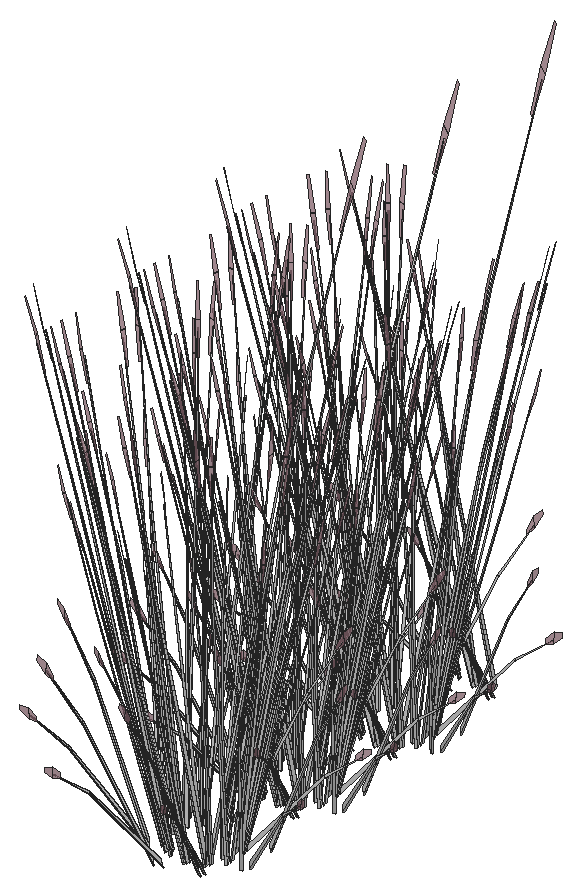
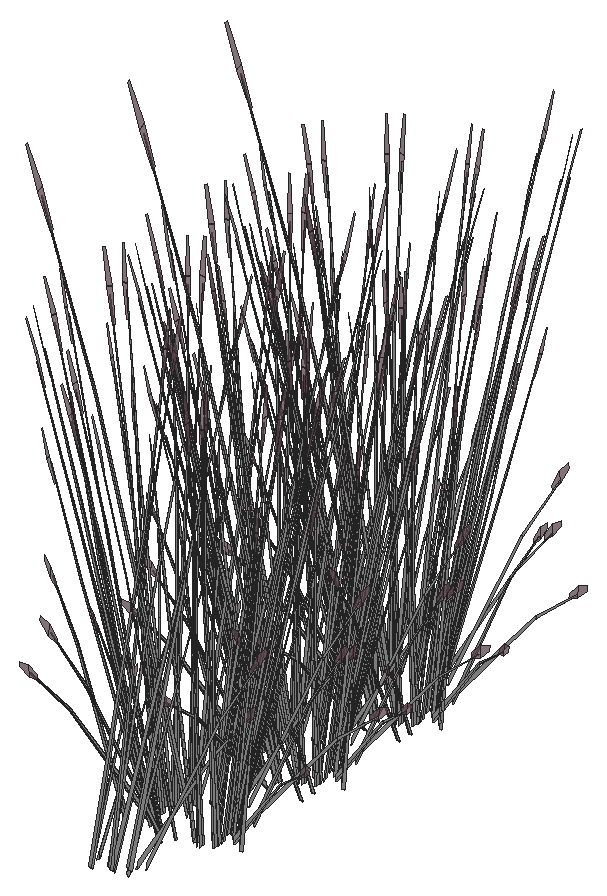
# SketchUp Ruby script. Lengths in inches.
U = 1.inch
M = Sketchup.active_model
def pt(a) = Geom::Point3d.new(a.map { |v| v * U })
def face(e, loops, mat)
  f = e.add_face(loops[0].map { |a| pt(a) })
  loops[1..].each { |l| e.add_face(l.map { |a| pt(a) }).erase! }
  f.material = f.back_material = mat if mat
  f
end
# faces: each face lists its corners as indices into pts; further lists are holes
def faces(e, pts, list, mat = nil) = list.each { |f| face(e, (f[0].is_a?(Array) ? f : [f]).map { |l| l.map { |i| pts[i] } }, mat) }
# xy, xz, yz: faces in a plane at the given z, y or x. An outline is a flat list of corners, or four numbers for a rectangle; further outlines are holes
def ring(l) = l.size == 4 ? [[l[0], l[1]], [l[2], l[1]], [l[2], l[3]], [l[0], l[3]]] : l.each_slice(2).to_a
def flat(e, list, mat, &to3) = list.each { |f| face(e, (f[0].is_a?(Array) ? f : [f]).map { |l| ring(l).map { |u, v| to3.(u, v) } }, mat) }
def xy(e, z, list, mat = nil) = flat(e, list, mat) { |x, y| [x, y, z] }
def xz(e, y, list, mat = nil) = flat(e, list, mat) { |x, z| [x, y, z] }
def yz(e, x, list, mat = nil) = flat(e, list, mat) { |y, z| [x, y, z] }
def lines(e, pts, list) = list.each { |a, b| e.add_line(pt(pts[a]), pt(pts[b])) }
# prism: a flat outline (further loops are holes) pulled along v
def prism(e, loops, v, mat = nil)
  f = face(e, loops, mat); d = Geom::Vector3d.new(v.map { |x| x * U })
  f.pushpull(f.normal.samedirection?(d) ? d.length : -d.length)
end
def box(e, o, s, mat = nil) = prism(e, [[o, [o[0] + s[0], o[1], o[2]], [o[0] + s[0], o[1] + s[1], o[2]], [o[0], o[1] + s[1], o[2]]]], [0, 0, s[2]], mat)
def at(x, y, z, deg = 0) = Geom::Transformation.translation(pt([x, y, z])) * Geom::Transformation.rotation(ORIGIN, Z_AXIS, deg.degrees)
def axes(o, x, y, z) = Geom::Transformation.new([*x, 0, *y, 0, *z, 0, *pt(o).to_a, 1])
def part(name) = M.definitions.add(name)
# library, detail: a bought-in or finely detailed component or shape, given as its bounding box
def library(name, o, s) = part(name).tap { |d| box(d.entities, o, s) }
def detail(e, o, s) = box(e.add_group.entities, o, s)
def put(e, d, t, mat = nil) = e.add_instance(d, t).tap { |i| i.material = mat if mat }
def group(e, t, mat = nil) = e.add_group.tap { |g| g.transformation = t; g.material = mat if mat }.entities
root = M.entities
M.materials.add("LightPink_Translucent").color = [144, 107, 117]
M.materials["LightPink_Translucent"].alpha = 0.75
M.materials.add("[_0053_Ivory_]").color = [200, 200, 200]
c1 = part("blade")
p = [[2.15,0.21,22],[0,0.17,0],[0.09,0.45,0],[2.18,0.31,22],[2.29,0.31,22],[0.38,0.45,0],
  [2.48,0.24,33],[2.49,0.24,33],[2.48,0.22,33]]
faces(c1.entities,p,[[0,1,2,3],[4,5,2,3],[6,3,4,7],[8,0,3,6]])
c2 = part("seeds")
p = [[0.3,-0.1,1.38],[-0.01,-0.03,1.59],[-0.01,-0.03,0.03],[0.14,-0.07,-0.07],[0.29,-0.03,3],[0.15,0.01,3.11]]
faces(c2.entities,p,[[0,1,2,3],[1,0,4,5]],"LightPink_Translucent")
c3 = part("blade with seeds")
put(c3.entities,c1,at(0,0,0))
put(c3.entities,c2,axes([2.4,0.25,30.99],[1.5799,-0.05474,1.17369],[-0.12525,1.92788,0.29478],[-0.07173,-0.02425,1.56792]))
put(root,c3,axes([631.55,280.53,256.37],[-0.0929,-0.08817,1.74944],[-0.61994,0.0559,-0.27667],[-0.09894,-0.21089,0.14031]),"[_0053_Ivory_]")
put(root,c3,axes([634.33,281.61,256.37],[-0.00586,-0.12516,1.74944],[-0.49517,-0.36172,-0.27667],[0.07656,-0.21927,0.14031]),"[_0053_Ivory_]")
put(root,c3,axes([634.2,281.16,256.36],[-0.06168,0.04803,1.77383],[-0.60432,-0.16205,-0.16761],[-0.02188,-0.20961,0.31391]),"[_0053_Ivory_]")
put(root,c3,axes([630.91,280.24,256.36],[-0.01133,0.07538,1.77383],[-0.55883,0.27355,-0.16761],[-0.16445,-0.13983,0.31391]),"[_0053_Ivory_]")
put(root,c3,axes([630.79,281.58,256.75],[0.67657,-0.16163,0.53763],[0.11742,0.63404,0.4433],[-0.15912,-0.18687,1.11249]),"[_0053_Ivory_]")
put(root,c3,axes([632.32,281.7,256.39],[0.59846,0.1644,0.48003],[-0.20464,0.54049,0.3958],[-0.03596,-0.21255,0.9933]),"[_0053_Ivory_]")
put(root,c3,axes([632.49,281.89,256.6875],[-0.59433,0.29278,-0.1216],[-0.29207,-0.51964,-0.67495],[-0.07842,-0.21898,1.02557]),"[_0053_Ivory_]")
put(root,c3,axes([633.72,282.55,256.6875],[-0.6675,-0.03116,-0.1216],[0.01824,-0.58993,-0.67495],[0.04637,-0.2272,1.02557]),"[_0053_Ivory_]")
put(root,c3,axes([632.48,281.65,256.38],[0.44753,-0.21372,0.0643],[0.21905,0.38973,0.50621],[-0.04322,-0.1718,0.77189]),"[_0053_Ivory_]")
put(root,c3,axes([630.94,281.71,256.38],[0.27604,-0.39948,0.0643],[0.39309,0.23258,0.50621],[-0.12709,-0.12808,0.77189]),"[_0053_Ivory_]")
put(root,c3,axes([632.31,282.09,256.7],[-0.1831,0.48359,0.35414],[-0.53419,-0.14105,-0.4572],[-0.04898,-0.1947,0.87481]),"[_0053_Ivory_]")
put(root,c3,axes([633.68,282.3,256.39],[0.43249,0.42907,0.48003],[-0.45929,0.37004,0.3958],[0.07978,-0.2013,0.9933]),"[_0053_Ivory_]")
put(root,c3,axes([631.07,281.67,257.08],[-0.40534,0.60286,-0.13619],[-0.58702,-0.34732,-0.75594],[-0.20405,-0.17032,1.14864]),"[_0053_Ivory_]")
put(root,c3,axes([633.84,282.34,256.38],[0.49911,0.0293,0.0643],[-0.01368,0.44245,0.50621],[0.05223,-0.16948,0.77189]),"[_0053_Ivory_]")
put(root,c3,axes([633.46,282.64,256.7],[-0.41095,0.33109,0.35414],[-0.38901,-0.37805,-0.4572],[0.05919,-0.19208,0.87481]),"[_0053_Ivory_]")
put(root,c3,axes([629.51,281.5,256.37],[-0.13068,-0.00444,1.74944],[-0.41604,0.44388,-0.27667],[-0.22198,-0.0907,0.14031]),"[_0053_Ivory_]")
put(root,c3,axes([634.45,283.71,256.6875],[-0.56181,-0.34675,-0.1216],[0.32367,-0.50216,-0.67495],[0.15873,-0.17455,1.02557]),"[_0053_Ivory_]")
put(root,c3,axes([631.03,282.17,256.7],[0.0938,0.50652,0.35414],[-0.53623,0.13375,-0.4572],[-0.14403,-0.14515,0.87481]),"[_0053_Ivory_]")
put(root,c3,axes([629.42,282.5,256.75],[0.50157,-0.46409,0.53763],[0.43258,0.49285,0.4433],[-0.23532,-0.08561,1.11249]),"[_0053_Ivory_]")
put(root,c3,axes([635.83,283.56,256.36],[-0.07933,-0.00478,1.77383],[-0.32942,-0.51175,-0.16761],[0.13229,-0.16826,0.31391]),"[_0053_Ivory_]")
put(root,c3,axes([629.65,282.5,256.38],[0.03058,-0.47819,0.0643],[0.4618,0.01311,0.50621],[-0.1769,-0.05004,0.77189]),"[_0053_Ivory_]")
put(root,c3,axes([634.18,283.66,256.7],[-0.52868,0.08987,0.35414],[-0.1396,-0.51376,-0.4572],[0.1515,-0.13799,0.87481]),"[_0053_Ivory_]")
put(root,c3,axes([634.66,283.58,256.38],[0.41695,0.26447,0.0643],[-0.24275,0.37662,0.50621],[0.13368,-0.12176,0.77189]),"[_0053_Ivory_]")
put(root,c3,axes([634.54,283.47,256.39],[0.15063,0.57876,0.48003],[-0.59087,0.10045,0.3958],[0.17414,-0.13612,0.9933]),"[_0053_Ivory_]")
put(root,c3,axes([636.13,284.17,256.37],[0.08428,-0.09579,1.74944],[-0.10787,-0.58756,-0.27667],[0.21147,-0.1114,0.14031]),"[_0053_Ivory_]")
put(root,c3,axes([629.01,281.875,256.36],[0.04503,0.06276,1.77383],[-0.21706,0.56413,-0.16761],[-0.21983,0.00408,0.31391]),"[_0053_Ivory_]")
put(root,c3,axes([629.96,282.86,256.7],[0.34557,0.39372,0.35414],[-0.39459,0.37271,-0.4572],[-0.20048,-0.05671,0.87481]),"[_0053_Ivory_]")
put(root,c3,axes([629.87,282.61,256.6875],[-0.03252,0.63953,-0.1216],[-0.61574,-0.01748,-0.67495],[-0.23714,-0.04442,1.02557]),"[_0053_Ivory_]")
put(root,c3,axes([634.47,285.0625,256.6875],[-0.30559,-0.56943,-0.1216],[0.54237,-0.27983,-0.67495],[0.22856,-0.07513,1.02557]),"[_0053_Ivory_]")
put(root,c3,axes([634.26,284.89,256.7],[-0.50475,-0.17543,0.35414],[0.14722,-0.5118,-0.4572],[0.20322,-0.04693,0.87481]),"[_0053_Ivory_]")
put(root,c3,axes([628.98,283.95,256.39],[0.17159,-0.57338,0.48003],[0.56413,0.19607,0.3958],[-0.22185,0.03446,0.9933]),"[_0053_Ivory_]")
put(root,c3,axes([628.93,283.8,256.38],[-0.22307,-0.42878,0.0643],[0.40677,-0.20987,0.50621],[-0.17931,0.04141,0.77189]),"[_0053_Ivory_]")
put(root,c3,axes([634.72,285.05,256.38],[0.22307,0.42878,0.0643],[-0.40677,0.20987,0.50621],[0.17931,-0.04141,0.77189]),"[_0053_Ivory_]")
put(root,c3,axes([634.68,284.9,256.39],[-0.17159,0.57338,0.48003],[-0.56413,-0.19607,0.3958],[0.22185,-0.03446,0.9933]),"[_0053_Ivory_]")
put(root,c3,axes([629.39,283.96,256.7],[0.50475,0.17543,0.35414],[-0.14722,0.5118,-0.4572],[-0.20322,0.04693,0.87481]),"[_0053_Ivory_]")
put(root,c3,axes([635.6875,286.75,256.36],[-0.05492,-0.05505,1.77383],[0.12013,-0.59013,-0.16761],[0.21632,-0.0377,0.31391]),"[_0053_Ivory_]")
put(root,c3,axes([628.54,284.36,256.37],[-0.09918,0.08165,1.74944],[0.00844,0.59653,-0.27667],[-0.22734,0.07758,0.14031]),"[_0053_Ivory_]")
put(root,c3,axes([629.18,283.79,256.6875],[0.30559,0.56943,-0.1216],[-0.54237,0.27983,-0.67495],[-0.22856,0.07513,1.02557]),"[_0053_Ivory_]")
put(root,c3,axes([633.79,286.24,256.6875],[0.03252,-0.63953,-0.1216],[0.61574,0.01748,-0.67495],[0.23714,0.04442,1.02557]),"[_0053_Ivory_]")
put(root,c3,axes([633.69,285.99,256.7],[-0.34557,-0.39372,0.35414],[0.39459,-0.37271,-0.4572],[0.20048,0.05671,0.87481]),"[_0053_Ivory_]")
put(root,c3,axes([631.55,290.36,256.37],[-0.0929,-0.08817,1.74944],[-0.61994,0.0559,-0.27667],[-0.09894,-0.21089,0.14031]),"[_0053_Ivory_]")
put(root,c3,axes([634.32,285.86,256.37],[0.13029,-0.01064,1.74944],[0.35737,-0.48855,-0.27667],[0.23175,0.06449,0.14031]),"[_0053_Ivory_]")
put(root,c3,axes([629.11,285.38,256.39],[-0.15063,-0.57876,0.48003],[0.59087,-0.10045,0.3958],[-0.17414,0.13612,0.9933]),"[_0053_Ivory_]")
put(root,c3,axes([629,285.27,256.38],[-0.41695,-0.26447,0.0643],[0.24275,-0.37662,0.50621],[-0.13368,0.12176,0.77189]),"[_0053_Ivory_]")
put(root,c3,axes([634.33,291.45,256.37],[-0.00586,-0.12516,1.74944],[-0.49517,-0.36172,-0.27667],[0.07656,-0.21927,0.14031]),"[_0053_Ivory_]")
put(root,c3,axes([634.2,291,256.36],[-0.06168,0.04803,1.77383],[-0.60432,-0.16205,-0.16761],[-0.02188,-0.20961,0.31391]),"[_0053_Ivory_]")
put(root,c3,axes([629.48,285.1875,256.7],[0.52868,-0.08987,0.35414],[0.1396,0.51376,-0.4572],[-0.1515,0.13799,0.87481]),"[_0053_Ivory_]")
put(root,c3,axes([630.91,290.08,256.36],[-0.01133,0.07538,1.77383],[-0.55883,0.27355,-0.16761],[-0.16445,-0.13983,0.31391]),"[_0053_Ivory_]")
put(root,c3,axes([627.4375,284.96,256.36],[0.07751,0.01687,1.77383],[0.23978,0.55562,-0.16761],[-0.15867,0.14583,0.31391]),"[_0053_Ivory_]")
put(root,c3,axes([630.79,291.41,256.75],[0.67657,-0.16163,0.53763],[0.11742,0.63404,0.4433],[-0.15912,-0.18687,1.11249]),"[_0053_Ivory_]")
put(root,c3,axes([634.01,286.35,256.38],[-0.03058,0.47819,0.0643],[-0.4618,-0.01311,0.50621],[0.1769,0.05004,0.77189]),"[_0053_Ivory_]")
put(root,c3,axes([632.32,291.53,256.39],[0.59846,0.1644,0.48003],[-0.20464,0.54049,0.3958],[-0.03596,-0.21255,0.9933]),"[_0053_Ivory_]")
put(root,c3,axes([632.49,291.73,256.6875],[-0.59433,0.29278,-0.1216],[-0.29207,-0.51964,-0.67495],[-0.07842,-0.21898,1.02557]),"[_0053_Ivory_]")
put(root,c3,axes([634.05,286.2,256.39],[-0.44783,0.41436,0.48003],[-0.38623,-0.44004,0.3958],[0.21011,0.07643,0.9933]),"[_0053_Ivory_]")
put(root,c3,axes([633.72,292.38,256.6875],[-0.6675,-0.03116,-0.1216],[0.01824,-0.58993,-0.67495],[0.04637,-0.2272,1.02557]),"[_0053_Ivory_]")
put(root,c3,axes([632.48,291.49,256.38],[0.44753,-0.21372,0.0643],[0.21905,0.38973,0.50621],[-0.04322,-0.1718,0.77189]),"[_0053_Ivory_]")
put(root,c3,axes([628.28,286.65,257.3],[0.53595,0.16786,-0.06488],[-0.16486,0.51664,-0.29416],[-0.08766,0.07844,0.97024]),"[_0053_Ivory_]")
put(root,c3,axes([632.625,286.68,256.7],[-0.0938,-0.50652,0.35414],[0.53623,-0.13375,-0.4572],[0.14403,0.14515,0.87481]),"[_0053_Ivory_]")
put(root,c3,axes([630.94,291.55,256.38],[0.27604,-0.39948,0.0643],[0.39309,0.23258,0.50621],[-0.12709,-0.12808,0.77189]),"[_0053_Ivory_]")
put(root,c3,axes([632.98,283.76,256.13],[-0.52482,-0.32674,1.38283],[0.55416,-0.50872,0.59665],[0.16933,0.30658,1.33663]),"[_0053_Ivory_]")
put(root,c3,axes([629.2,285.14,256.6875],[0.56181,0.34675,-0.1216],[-0.32367,0.50216,-0.67495],[-0.15873,0.17455,1.02557]),"[_0053_Ivory_]")
put(root,c3,axes([632.57,286.9375,256.6875],[0.36191,-0.53827,-0.1216],[0.52412,0.3101,-0.67495],[0.18219,0.15207,1.02557]),"[_0053_Ivory_]")
put(root,c3,axes([632.31,291.93,256.7],[-0.1831,0.48359,0.35414],[-0.53419,-0.14105,-0.4572],[-0.04898,-0.1947,0.87481]),"[_0053_Ivory_]")
put(root,c3,axes([633.68,292.13,256.39],[0.43249,0.42907,0.48003],[-0.45929,0.37004,0.3958],[0.07978,-0.2013,0.9933]),"[_0053_Ivory_]")
put(root,c3,axes([631.07,291.51,257.08],[-0.40534,0.60286,-0.13619],[-0.58702,-0.34732,-0.75594],[-0.20405,-0.17032,1.14864]),"[_0053_Ivory_]")
put(root,c3,axes([633.84,292.17,256.38],[0.49911,0.0293,0.0643],[-0.01368,0.44245,0.50621],[0.05223,-0.16948,0.77189]),"[_0053_Ivory_]")
put(root,c3,axes([630.1875,286.21,256.7],[0.41095,-0.33109,0.35414],[0.38901,0.37805,-0.4572],[-0.05919,0.19208,0.87481]),"[_0053_Ivory_]")
put(root,c3,axes([632.1,287.39,256.36],[0.0018,-0.07613,1.77383],[0.52048,-0.3359,-0.16761],[0.18079,0.11989,0.31391]),"[_0053_Ivory_]")
put(root,c3,axes([633.46,292.47,256.7],[-0.41095,0.33109,0.35414],[-0.38901,-0.37805,-0.4572],[0.05919,-0.19208,0.87481]),"[_0053_Ivory_]")
put(root,c3,axes([629.82,286.51,256.38],[-0.49911,-0.0293,0.0643],[0.01368,-0.44245,0.50621],[-0.05223,0.16948,0.77189]),"[_0053_Ivory_]")
put(root,c3,axes([629.98,286.55,256.39],[-0.43249,-0.42907,0.48003],[0.45929,-0.37004,0.3958],[-0.07978,0.2013,0.9933]),"[_0053_Ivory_]")
put(root,c3,axes([631.34,286.76,256.7],[0.1831,-0.48359,0.35414],[0.53419,0.14105,-0.4572],[0.04898,0.1947,0.87481]),"[_0053_Ivory_]")
put(root,c3,axes([629.51,291.34,256.37],[-0.13068,-0.00444,1.74944],[-0.41604,0.44388,-0.27667],[-0.22198,-0.0907,0.14031]),"[_0053_Ivory_]")
put(root,c3,axes([634.45,293.54,256.6875],[-0.56181,-0.34675,-0.1216],[0.32367,-0.50216,-0.67495],[0.15873,-0.17455,1.02557]),"[_0053_Ivory_]")
put(root,c3,axes([632.71,287.14,256.38],[-0.27604,0.39948,0.0643],[-0.39309,-0.23258,0.50621],[0.12709,0.12808,0.77189]),"[_0053_Ivory_]")
put(root,c3,axes([632.06,288.48,257.3],[0.4197,-0.36076,-0.06488],[0.38456,0.39511,-0.29416],[0.02707,0.11196,0.97024]),"[_0053_Ivory_]")
put(root,c3,axes([632.82,287.02,256.39],[-0.60408,0.14432,0.48003],[-0.10484,-0.56611,0.3958],[0.14207,0.16684,0.9933]),"[_0053_Ivory_]")
put(root,c3,axes([631.03,292.01,256.7],[0.0938,0.50652,0.35414],[-0.53623,0.13375,-0.4572],[-0.14403,-0.14515,0.87481]),"[_0053_Ivory_]")
put(root,c3,axes([629.42,292.34,256.75],[0.50157,-0.46409,0.53763],[0.43258,0.49285,0.4433],[-0.23532,-0.08561,1.11249]),"[_0053_Ivory_]")
put(root,c3,axes([635.83,293.39,256.36],[-0.07933,-0.00478,1.77383],[-0.32942,-0.51175,-0.16761],[0.13229,-0.16826,0.31391]),"[_0053_Ivory_]")
put(root,c3,axes([631.18,287.2,256.38],[-0.44753,0.21372,0.0643],[-0.21905,-0.38973,0.50621],[0.04322,0.1718,0.77189]),"[_0053_Ivory_]")
put(root,c3,axes([628.56,286.58,256.37],[-0.0151,0.12444,1.74944],[0.42844,0.43292,-0.27667],[-0.11216,0.20472,0.14031]),"[_0053_Ivory_]")
put(root,c3,axes([629.93,286.3,257.05],[0.6675,0.03116,-0.13498],[-0.01824,0.58993,-0.74919],[-0.04637,0.2272,1.13838]),"[_0053_Ivory_]")
put(root,c3,axes([631.16,286.96,256.6875],[0.59433,-0.29278,-0.1216],[0.29207,0.51964,-0.67495],[0.07842,0.21898,1.02557]),"[_0053_Ivory_]")
put(root,c3,axes([631.33,287.15,256.72],[-0.59846,-0.1644,0.53283],[0.20464,-0.54049,0.43934],[0.03596,0.21255,1.10256]),"[_0053_Ivory_]")
put(root,c3,axes([629.65,292.34,256.38],[0.03058,-0.47819,0.0643],[0.4618,0.01311,0.50621],[-0.1769,-0.05004,0.77189]),"[_0053_Ivory_]")
put(root,c3,axes([634.18,293.5,256.7],[-0.52868,0.08987,0.35414],[-0.1396,-0.51376,-0.4572],[0.1515,-0.13799,0.87481]),"[_0053_Ivory_]")
put(root,c3,axes([628.51,287.86,256.36],[0.0689,-0.03797,1.77383],[0.5695,0.25254,-0.16761],[-0.01338,0.21027,0.31391]),"[_0053_Ivory_]")
put(root,c3,axes([634.66,293.42,256.38],[0.41695,0.26447,0.0643],[-0.24275,0.37662,0.50621],[0.13368,-0.12176,0.77189]),"[_0053_Ivory_]")
put(root,c3,axes([634.54,293.3,256.39],[0.15063,0.57876,0.48003],[-0.59087,0.10045,0.3958],[0.17414,-0.13612,0.9933]),"[_0053_Ivory_]")
put(root,c3,axes([636.13,294.01,256.37],[0.08428,-0.09579,1.74944],[-0.10787,-0.58756,-0.27667],[0.21147,-0.1114,0.14031]),"[_0053_Ivory_]")
put(root,c3,axes([629.01,291.71,256.36],[0.04503,0.06276,1.77383],[-0.21706,0.56413,-0.16761],[-0.21983,0.00408,0.31391]),"[_0053_Ivory_]")
put(root,c3,axes([629.96,292.69,256.7],[0.34557,0.39372,0.35414],[-0.39459,0.37271,-0.4572],[-0.20048,-0.05671,0.87481]),"[_0053_Ivory_]")
put(root,c3,axes([631.02,288.125,256.37],[0.07699,0.10127,1.74944],[0.6213,0.03978,-0.27667],[0.06248,0.22333,0.14031]),"[_0053_Ivory_]")
put(root,c3,axes([629.87,292.44,256.6875],[-0.03252,0.63953,-0.1216],[-0.61574,-0.01748,-0.67495],[-0.23714,-0.04442,1.02557]),"[_0053_Ivory_]")
put(root,c3,axes([634.47,294.9,256.6875],[-0.30559,-0.56943,-0.1216],[0.54237,-0.27983,-0.67495],[0.22856,-0.07513,1.02557]),"[_0053_Ivory_]")
put(root,c3,axes([634.26,294.73,256.7],[-0.50475,-0.17543,0.35414],[0.14722,-0.5118,-0.4572],[0.20322,-0.04693,0.87481]),"[_0053_Ivory_]")
put(root,c3,axes([628.98,293.79,256.39],[0.17159,-0.57338,0.48003],[0.56413,0.19607,0.3958],[-0.22185,0.03446,0.9933]),"[_0053_Ivory_]")
put(root,c3,axes([628.93,293.64,256.38],[-0.22307,-0.42878,0.0643],[0.40677,-0.20987,0.50621],[-0.17931,0.04141,0.77189]),"[_0053_Ivory_]")
put(root,c3,axes([634.72,294.88,256.38],[0.22307,0.42878,0.0643],[-0.40677,0.20987,0.50621],[0.17931,-0.04141,0.77189]),"[_0053_Ivory_]")
put(root,c3,axes([634.68,294.73,256.39],[-0.17159,0.57338,0.48003],[-0.56413,-0.19607,0.3958],[0.22185,-0.03446,0.9933]),"[_0053_Ivory_]")
put(root,c3,axes([629.39,293.8,256.7],[0.50475,0.17543,0.35414],[-0.14722,0.5118,-0.4572],[-0.20322,0.04693,0.87481]),"[_0053_Ivory_]")
put(root,c3,axes([635.6875,296.59,256.36],[-0.05492,-0.05505,1.77383],[0.12013,-0.59013,-0.16761],[0.21632,-0.0377,0.31391]),"[_0053_Ivory_]")
put(root,c3,axes([628.54,294.19,256.37],[-0.09918,0.08165,1.74944],[0.00844,0.59653,-0.27667],[-0.22734,0.07758,0.14031]),"[_0053_Ivory_]")
put(root,c3,axes([629.18,293.625,256.6875],[0.30559,0.56943,-0.1216],[-0.54237,0.27983,-0.67495],[-0.22856,0.07513,1.02557]),"[_0053_Ivory_]")
put(root,c3,axes([633.79,296.08,256.6875],[0.03252,-0.63953,-0.1216],[0.61574,0.01748,-0.67495],[0.23714,0.04442,1.02557]),"[_0053_Ivory_]")
put(root,c3,axes([633.69,295.83,256.7],[-0.34557,-0.39372,0.35414],[0.39459,-0.37271,-0.4572],[0.20048,0.05671,0.87481]),"[_0053_Ivory_]")
put(root,c3,axes([631.55,300.66,256.37],[-0.0929,-0.08817,1.74944],[-0.61994,0.0559,-0.27667],[-0.09894,-0.21089,0.14031]),"[_0053_Ivory_]")
put(root,c3,axes([634.32,295.7,256.37],[0.13029,-0.01064,1.74944],[0.35737,-0.48855,-0.27667],[0.23175,0.06449,0.14031]),"[_0053_Ivory_]")
put(root,c3,axes([629.11,295.22,256.39],[-0.15063,-0.57876,0.48003],[0.59087,-0.10045,0.3958],[-0.17414,0.13612,0.9933]),"[_0053_Ivory_]")
put(root,c3,axes([629,295.11,256.38],[-0.41695,-0.26447,0.0643],[0.24275,-0.37662,0.50621],[-0.13368,0.12176,0.77189]),"[_0053_Ivory_]")
put(root,c3,axes([629.48,295.03,256.7],[0.52868,-0.08987,0.35414],[0.1396,0.51376,-0.4572],[-0.1515,0.13799,0.87481]),"[_0053_Ivory_]")
put(root,c3,axes([634.33,301.74,256.37],[-0.00586,-0.12516,1.74944],[-0.49517,-0.36172,-0.27667],[0.07656,-0.21927,0.14031]),"[_0053_Ivory_]")
put(root,c3,axes([634.2,301.29,256.36],[-0.06168,0.04803,1.77383],[-0.60432,-0.16205,-0.16761],[-0.02188,-0.20961,0.31391]),"[_0053_Ivory_]")
put(root,c3,axes([627.4375,294.8,256.36],[0.07751,0.01687,1.77383],[0.23978,0.55562,-0.16761],[-0.15867,0.14583,0.31391]),"[_0053_Ivory_]")
put(root,c3,axes([634.01,296.1875,256.38],[-0.03058,0.47819,0.0643],[-0.4618,-0.01311,0.50621],[0.1769,0.05004,0.77189]),"[_0053_Ivory_]")
put(root,c3,axes([634.05,296.03,256.39],[-0.44783,0.41436,0.48003],[-0.38623,-0.44004,0.3958],[0.21011,0.07643,0.9933]),"[_0053_Ivory_]")
put(root,c3,axes([630.91,300.37,256.36],[-0.01133,0.07538,1.77383],[-0.55883,0.27355,-0.16761],[-0.16445,-0.13983,0.31391]),"[_0053_Ivory_]")
put(root,c3,axes([630.79,301.71,256.75],[0.67657,-0.16163,0.53763],[0.11742,0.63404,0.4433],[-0.15912,-0.18687,1.11249]),"[_0053_Ivory_]")
put(root,c3,axes([628.28,296.49,257.3],[0.53595,0.16786,-0.06488],[-0.16486,0.51664,-0.29416],[-0.08766,0.07844,0.97024]),"[_0053_Ivory_]")
put(root,c3,axes([632.32,301.83,256.39],[0.59846,0.1644,0.48003],[-0.20464,0.54049,0.3958],[-0.03596,-0.21255,0.9933]),"[_0053_Ivory_]")
put(root,c3,axes([632.49,302.02,256.6875],[-0.59433,0.29278,-0.1216],[-0.29207,-0.51964,-0.67495],[-0.07842,-0.21898,1.02557]),"[_0053_Ivory_]")
put(root,c3,axes([632.625,296.51,256.7],[-0.0938,-0.50652,0.35414],[0.53623,-0.13375,-0.4572],[0.14403,0.14515,0.87481]),"[_0053_Ivory_]")
put(root,c3,axes([633.72,302.68,256.6875],[-0.6675,-0.03116,-0.1216],[0.01824,-0.58993,-0.67495],[0.04637,-0.2272,1.02557]),"[_0053_Ivory_]")
put(root,c3,axes([632.48,301.79,256.38],[0.44753,-0.21372,0.0643],[0.21905,0.38973,0.50621],[-0.04322,-0.1718,0.77189]),"[_0053_Ivory_]")
put(root,c3,axes([632.98,293.6,256.13],[-0.52482,-0.32674,1.38283],[0.55416,-0.50872,0.59665],[0.16933,0.30658,1.33663]),"[_0053_Ivory_]")
put(root,c3,axes([629.2,294.98,256.6875],[0.56181,0.34675,-0.1216],[-0.32367,0.50216,-0.67495],[-0.15873,0.17455,1.02557]),"[_0053_Ivory_]")
put(root,c3,axes([632.57,296.78,256.6875],[0.36191,-0.53827,-0.1216],[0.52412,0.3101,-0.67495],[0.18219,0.15207,1.02557]),"[_0053_Ivory_]")
put(root,c3,axes([630.94,301.85,256.38],[0.27604,-0.39948,0.0643],[0.39309,0.23258,0.50621],[-0.12709,-0.12808,0.77189]),"[_0053_Ivory_]")
put(root,c3,axes([630.1875,296.05,256.7],[0.41095,-0.33109,0.35414],[0.38901,0.37805,-0.4572],[-0.05919,0.19208,0.87481]),"[_0053_Ivory_]")
put(root,c3,axes([632.1,297.22,256.36],[0.0018,-0.07613,1.77383],[0.52048,-0.3359,-0.16761],[0.18079,0.11989,0.31391]),"[_0053_Ivory_]")
put(root,c3,axes([629.82,296.35,256.38],[-0.49911,-0.0293,0.0643],[0.01368,-0.44245,0.50621],[-0.05223,0.16948,0.77189]),"[_0053_Ivory_]")
put(root,c3,axes([629.98,296.39,256.39],[-0.43249,-0.42907,0.48003],[0.45929,-0.37004,0.3958],[-0.07978,0.2013,0.9933]),"[_0053_Ivory_]")
put(root,c3,axes([632.31,302.22,256.7],[-0.1831,0.48359,0.35414],[-0.53419,-0.14105,-0.4572],[-0.04898,-0.1947,0.87481]),"[_0053_Ivory_]")
put(root,c3,axes([631.34,296.59,256.7],[0.1831,-0.48359,0.35414],[0.53419,0.14105,-0.4572],[0.04898,0.1947,0.87481]),"[_0053_Ivory_]")
put(root,c3,axes([633.68,302.43,256.39],[0.43249,0.42907,0.48003],[-0.45929,0.37004,0.3958],[0.07978,-0.2013,0.9933]),"[_0053_Ivory_]")
put(root,c3,axes([631.07,301.8,257.08],[-0.40534,0.60286,-0.13619],[-0.58702,-0.34732,-0.75594],[-0.20405,-0.17032,1.14864]),"[_0053_Ivory_]")
put(root,c3,axes([633.84,302.47,256.38],[0.49911,0.0293,0.0643],[-0.01368,0.44245,0.50621],[0.05223,-0.16948,0.77189]),"[_0053_Ivory_]")
put(root,c3,axes([633.46,302.77,256.7],[-0.41095,0.33109,0.35414],[-0.38901,-0.37805,-0.4572],[0.05919,-0.19208,0.87481]),"[_0053_Ivory_]")
put(root,c3,axes([632.71,296.97,256.38],[-0.27604,0.39948,0.0643],[-0.39309,-0.23258,0.50621],[0.12709,0.12808,0.77189]),"[_0053_Ivory_]")
put(root,c3,axes([632.06,298.32,257.3],[0.4197,-0.36076,-0.06488],[0.38456,0.39511,-0.29416],[0.02707,0.11196,0.97024]),"[_0053_Ivory_]")
put(root,c3,axes([632.82,296.86,256.39],[-0.60408,0.14432,0.48003],[-0.10484,-0.56611,0.3958],[0.14207,0.16684,0.9933]),"[_0053_Ivory_]")
put(root,c3,axes([629.51,301.63,256.37],[-0.13068,-0.00444,1.74944],[-0.41604,0.44388,-0.27667],[-0.22198,-0.0907,0.14031]),"[_0053_Ivory_]")
put(root,c3,axes([634.45,303.84,256.6875],[-0.56181,-0.34675,-0.1216],[0.32367,-0.50216,-0.67495],[0.15873,-0.17455,1.02557]),"[_0053_Ivory_]")
put(root,c3,axes([631.18,297.03,256.38],[-0.44753,0.21372,0.0643],[-0.21905,-0.38973,0.50621],[0.04322,0.1718,0.77189]),"[_0053_Ivory_]")
put(root,c3,axes([628.56,296.42,256.37],[-0.0151,0.12444,1.74944],[0.42844,0.43292,-0.27667],[-0.11216,0.20472,0.14031]),"[_0053_Ivory_]")
put(root,c3,axes([629.93,296.14,257.05],[0.6675,0.03116,-0.13498],[-0.01824,0.58993,-0.74919],[-0.04637,0.2272,1.13838]),"[_0053_Ivory_]")
put(root,c3,axes([631.03,302.3,256.7],[0.0938,0.50652,0.35414],[-0.53623,0.13375,-0.4572],[-0.14403,-0.14515,0.87481]),"[_0053_Ivory_]")
put(root,c3,axes([631.16,296.8,256.6875],[0.59433,-0.29278,-0.1216],[0.29207,0.51964,-0.67495],[0.07842,0.21898,1.02557]),"[_0053_Ivory_]")
put(root,c3,axes([631.33,296.99,256.72],[-0.59846,-0.1644,0.53283],[0.20464,-0.54049,0.43934],[0.03596,0.21255,1.10256]),"[_0053_Ivory_]")
put(root,c3,axes([629.42,302.63,256.75],[0.50157,-0.46409,0.53763],[0.43258,0.49285,0.4433],[-0.23532,-0.08561,1.11249]),"[_0053_Ivory_]")
put(root,c3,axes([635.83,303.6875,256.36],[-0.07933,-0.00478,1.77383],[-0.32942,-0.51175,-0.16761],[0.13229,-0.16826,0.31391]),"[_0053_Ivory_]")
put(root,c3,axes([629.65,302.63,256.38],[0.03058,-0.47819,0.0643],[0.4618,0.01311,0.50621],[-0.1769,-0.05004,0.77189]),"[_0053_Ivory_]")
put(root,c3,axes([634.18,303.79,256.7],[-0.52868,0.08987,0.35414],[-0.1396,-0.51376,-0.4572],[0.1515,-0.13799,0.87481]),"[_0053_Ivory_]")
put(root,c3,axes([628.51,297.7,256.36],[0.0689,-0.03797,1.77383],[0.5695,0.25254,-0.16761],[-0.01338,0.21027,0.31391]),"[_0053_Ivory_]")
put(root,c3,axes([634.66,303.71,256.38],[0.41695,0.26447,0.0643],[-0.24275,0.37662,0.50621],[0.13368,-0.12176,0.77189]),"[_0053_Ivory_]")
put(root,c3,axes([634.54,303.6,256.39],[0.15063,0.57876,0.48003],[-0.59087,0.10045,0.3958],[0.17414,-0.13612,0.9933]),"[_0053_Ivory_]")
put(root,c3,axes([636.13,304.3,256.37],[0.08428,-0.09579,1.74944],[-0.10787,-0.58756,-0.27667],[0.21147,-0.1114,0.14031]),"[_0053_Ivory_]")
put(root,c3,axes([631.02,297.96,256.37],[0.07699,0.10127,1.74944],[0.6213,0.03978,-0.27667],[0.06248,0.22333,0.14031]),"[_0053_Ivory_]")
put(root,c3,axes([629.01,302.01,256.36],[0.04503,0.06276,1.77383],[-0.21706,0.56413,-0.16761],[-0.21983,0.00408,0.31391]),"[_0053_Ivory_]")
put(root,c3,axes([629.96,302.99,256.7],[0.34557,0.39372,0.35414],[-0.39459,0.37271,-0.4572],[-0.20048,-0.05671,0.87481]),"[_0053_Ivory_]")
put(root,c3,axes([629.87,302.74,256.6875],[-0.03252,0.63953,-0.1216],[-0.61574,-0.01748,-0.67495],[-0.23714,-0.04442,1.02557]),"[_0053_Ivory_]")
put(root,c3,axes([634.47,305.19,256.6875],[-0.30559,-0.56943,-0.1216],[0.54237,-0.27983,-0.67495],[0.22856,-0.07513,1.02557]),"[_0053_Ivory_]")
put(root,c3,axes([634.26,305.02,256.7],[-0.50475,-0.17543,0.35414],[0.14722,-0.5118,-0.4572],[0.20322,-0.04693,0.87481]),"[_0053_Ivory_]")
put(root,c3,axes([628.98,304.09,256.39],[0.17159,-0.57338,0.48003],[0.56413,0.19607,0.3958],[-0.22185,0.03446,0.9933]),"[_0053_Ivory_]")
put(root,c3,axes([628.93,303.93,256.38],[-0.22307,-0.42878,0.0643],[0.40677,-0.20987,0.50621],[-0.17931,0.04141,0.77189]),"[_0053_Ivory_]")
put(root,c3,axes([634.72,305.18,256.38],[0.22307,0.42878,0.0643],[-0.40677,0.20987,0.50621],[0.17931,-0.04141,0.77189]),"[_0053_Ivory_]")
put(root,c3,axes([634.68,305.03,256.39],[-0.17159,0.57338,0.48003],[-0.56413,-0.19607,0.3958],[0.22185,-0.03446,0.9933]),"[_0053_Ivory_]")
put(root,c3,axes([629.39,304.09,256.7],[0.50475,0.17543,0.35414],[-0.14722,0.5118,-0.4572],[-0.20322,0.04693,0.87481]),"[_0053_Ivory_]")
put(root,c3,axes([635.6875,306.88,256.36],[-0.05492,-0.05505,1.77383],[0.12013,-0.59013,-0.16761],[0.21632,-0.0377,0.31391]),"[_0053_Ivory_]")
put(root,c3,axes([628.54,304.49,256.37],[-0.09918,0.08165,1.74944],[0.00844,0.59653,-0.27667],[-0.22734,0.07758,0.14031]),"[_0053_Ivory_]")
put(root,c3,axes([629.18,303.92,256.6875],[0.30559,0.56943,-0.1216],[-0.54237,0.27983,-0.67495],[-0.22856,0.07513,1.02557]),"[_0053_Ivory_]")
put(root,c3,axes([633.79,306.375,256.6875],[0.03252,-0.63953,-0.1216],[0.61574,0.01748,-0.67495],[0.23714,0.04442,1.02557]),"[_0053_Ivory_]")
put(root,c3,axes([633.69,306.125,256.7],[-0.34557,-0.39372,0.35414],[0.39459,-0.37271,-0.4572],[0.20048,0.05671,0.87481]),"[_0053_Ivory_]")
put(root,c3,axes([634.32,305.99,256.37],[0.13029,-0.01064,1.74944],[0.35737,-0.48855,-0.27667],[0.23175,0.06449,0.14031]),"[_0053_Ivory_]")
put(root,c3,axes([631.55,311.05,256.37],[-0.0929,-0.08817,1.74944],[-0.61994,0.0559,-0.27667],[-0.09894,-0.21089,0.14031]),"[_0053_Ivory_]")
put(root,c3,axes([629.11,305.51,256.39],[-0.15063,-0.57876,0.48003],[0.59087,-0.10045,0.3958],[-0.17414,0.13612,0.9933]),"[_0053_Ivory_]")
put(root,c3,axes([629,305.4,256.38],[-0.41695,-0.26447,0.0643],[0.24275,-0.37662,0.50621],[-0.13368,0.12176,0.77189]),"[_0053_Ivory_]")
put(root,c3,axes([629.48,305.32,256.7],[0.52868,-0.08987,0.35414],[0.1396,0.51376,-0.4572],[-0.1515,0.13799,0.87481]),"[_0053_Ivory_]")
put(root,c3,axes([627.4375,305.09,256.36],[0.07751,0.01687,1.77383],[0.23978,0.55562,-0.16761],[-0.15867,0.14583,0.31391]),"[_0053_Ivory_]")
put(root,c3,axes([634.33,312.13,256.37],[-0.00586,-0.12516,1.74944],[-0.49517,-0.36172,-0.27667],[0.07656,-0.21927,0.14031]),"[_0053_Ivory_]")
put(root,c3,axes([634.2,311.68,256.36],[-0.06168,0.04803,1.77383],[-0.60432,-0.16205,-0.16761],[-0.02188,-0.20961,0.31391]),"[_0053_Ivory_]")
put(root,c3,axes([634.01,306.48,256.38],[-0.03058,0.47819,0.0643],[-0.4618,-0.01311,0.50621],[0.1769,0.05004,0.77189]),"[_0053_Ivory_]")
put(root,c3,axes([634.05,306.33,256.39],[-0.44783,0.41436,0.48003],[-0.38623,-0.44004,0.3958],[0.21011,0.07643,0.9933]),"[_0053_Ivory_]")
put(root,c3,axes([630.91,310.76,256.36],[-0.01133,0.07538,1.77383],[-0.55883,0.27355,-0.16761],[-0.16445,-0.13983,0.31391]),"[_0053_Ivory_]")
put(root,c3,axes([628.28,306.78,257.3],[0.53595,0.16786,-0.06488],[-0.16486,0.51664,-0.29416],[-0.08766,0.07844,0.97024]),"[_0053_Ivory_]")
put(root,c3,axes([630.79,312.1,256.75],[0.67657,-0.16163,0.53763],[0.11742,0.63404,0.4433],[-0.15912,-0.18687,1.11249]),"[_0053_Ivory_]")
put(root,c3,axes([632.625,306.81,256.7],[-0.0938,-0.50652,0.35414],[0.53623,-0.13375,-0.4572],[0.14403,0.14515,0.87481]),"[_0053_Ivory_]")
put(root,c3,axes([632.32,312.22,256.39],[0.59846,0.1644,0.48003],[-0.20464,0.54049,0.3958],[-0.03596,-0.21255,0.9933]),"[_0053_Ivory_]")
put(root,c3,axes([632.49,312.41,256.6875],[-0.59433,0.29278,-0.1216],[-0.29207,-0.51964,-0.67495],[-0.07842,-0.21898,1.02557]),"[_0053_Ivory_]")
put(root,c3,axes([633.72,313.07,256.6875],[-0.6675,-0.03116,-0.1216],[0.01824,-0.58993,-0.67495],[0.04637,-0.2272,1.02557]),"[_0053_Ivory_]")
put(root,c3,axes([632.48,312.18,256.38],[0.44753,-0.21372,0.0643],[0.21905,0.38973,0.50621],[-0.04322,-0.1718,0.77189]),"[_0053_Ivory_]")
put(root,c3,axes([632.98,303.9,256.13],[-0.52482,-0.32674,1.38283],[0.55416,-0.50872,0.59665],[0.16933,0.30658,1.33663]),"[_0053_Ivory_]")
put(root,c3,axes([629.2,305.27,256.6875],[0.56181,0.34675,-0.1216],[-0.32367,0.50216,-0.67495],[-0.15873,0.17455,1.02557]),"[_0053_Ivory_]")
put(root,c3,axes([632.57,307.07,256.6875],[0.36191,-0.53827,-0.1216],[0.52412,0.3101,-0.67495],[0.18219,0.15207,1.02557]),"[_0053_Ivory_]")
put(root,c3,axes([630.94,312.24,256.38],[0.27604,-0.39948,0.0643],[0.39309,0.23258,0.50621],[-0.12709,-0.12808,0.77189]),"[_0053_Ivory_]")
put(root,c3,axes([630.1875,306.34,256.7],[0.41095,-0.33109,0.35414],[0.38901,0.37805,-0.4572],[-0.05919,0.19208,0.87481]),"[_0053_Ivory_]")
put(root,c3,axes([632.1,307.52,256.36],[0.0018,-0.07613,1.77383],[0.52048,-0.3359,-0.16761],[0.18079,0.11989,0.31391]),"[_0053_Ivory_]")
put(root,c3,axes([629.82,306.64,256.38],[-0.49911,-0.0293,0.0643],[0.01368,-0.44245,0.50621],[-0.05223,0.16948,0.77189]),"[_0053_Ivory_]")
put(root,c3,axes([629.98,306.69,256.39],[-0.43249,-0.42907,0.48003],[0.45929,-0.37004,0.3958],[-0.07978,0.2013,0.9933]),"[_0053_Ivory_]")
put(root,c3,axes([631.34,306.89,256.7],[0.1831,-0.48359,0.35414],[0.53419,0.14105,-0.4572],[0.04898,0.1947,0.87481]),"[_0053_Ivory_]")
